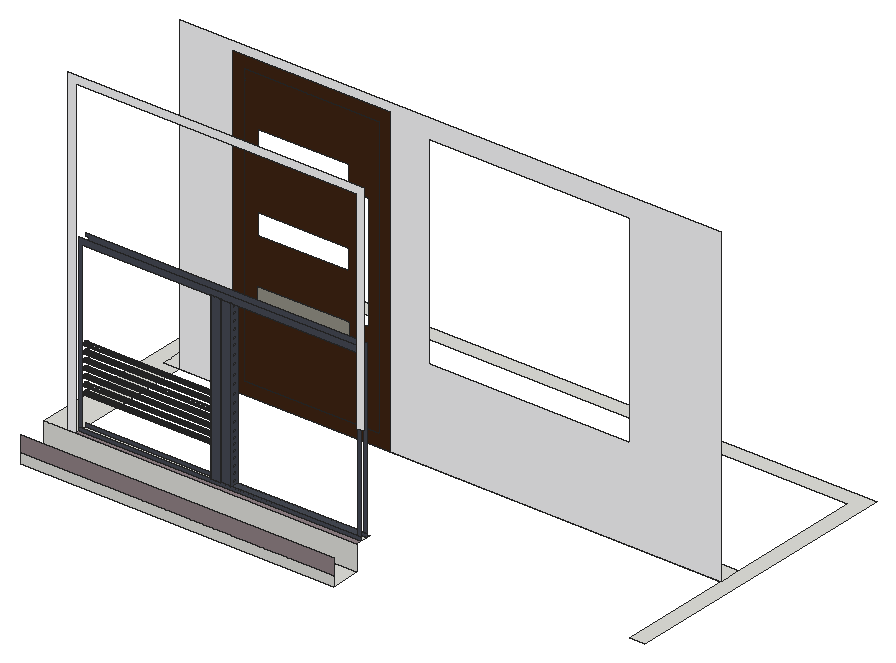
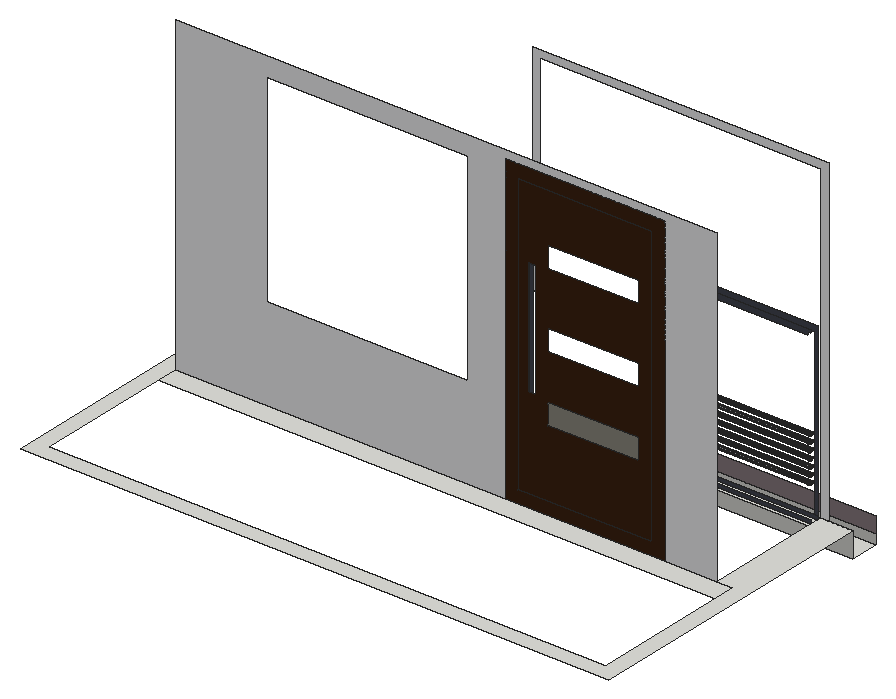
# SketchUp Ruby script. Lengths in inches.
U = 1.inch
M = Sketchup.active_model
def pt(a) = Geom::Point3d.new(a.map { |v| v * U })
def face(e, loops, mat)
  f = e.add_face(loops[0].map { |a| pt(a) })
  loops[1..].each { |l| e.add_face(l.map { |a| pt(a) }).erase! }
  f.material = f.back_material = mat if mat
  f
end
# faces: each face lists its corners as indices into pts; further lists are holes
def faces(e, pts, list, mat = nil) = list.each { |f| face(e, (f[0].is_a?(Array) ? f : [f]).map { |l| l.map { |i| pts[i] } }, mat) }
# xy, xz, yz: faces in a plane at the given z, y or x. An outline is a flat list of corners, or four numbers for a rectangle; further outlines are holes
def ring(l) = l.size == 4 ? [[l[0], l[1]], [l[2], l[1]], [l[2], l[3]], [l[0], l[3]]] : l.each_slice(2).to_a
def flat(e, list, mat, &to3) = list.each { |f| face(e, (f[0].is_a?(Array) ? f : [f]).map { |l| ring(l).map { |u, v| to3.(u, v) } }, mat) }
def xy(e, z, list, mat = nil) = flat(e, list, mat) { |x, y| [x, y, z] }
def xz(e, y, list, mat = nil) = flat(e, list, mat) { |x, z| [x, y, z] }
def yz(e, x, list, mat = nil) = flat(e, list, mat) { |y, z| [x, y, z] }
def lines(e, pts, list) = list.each { |a, b| e.add_line(pt(pts[a]), pt(pts[b])) }
# prism: a flat outline (further loops are holes) pulled along v
def prism(e, loops, v, mat = nil)
  f = face(e, loops, mat); d = Geom::Vector3d.new(v.map { |x| x * U })
  f.pushpull(f.normal.samedirection?(d) ? d.length : -d.length)
end
def box(e, o, s, mat = nil) = prism(e, [[o, [o[0] + s[0], o[1], o[2]], [o[0] + s[0], o[1] + s[1], o[2]], [o[0], o[1] + s[1], o[2]]]], [0, 0, s[2]], mat)
def at(x, y, z, deg = 0) = Geom::Transformation.translation(pt([x, y, z])) * Geom::Transformation.rotation(ORIGIN, Z_AXIS, deg.degrees)
def axes(o, x, y, z) = Geom::Transformation.new([*x, 0, *y, 0, *z, 0, *pt(o).to_a, 1])
def part(name) = M.definitions.add(name)
# library, detail: a bought-in or finely detailed component or shape, given as its bounding box
def library(name, o, s) = part(name).tap { |d| box(d.entities, o, s) }
def detail(e, o, s) = box(e.add_group.entities, o, s)
def put(e, d, t, mat = nil) = e.add_instance(d, t).tap { |i| i.material = mat if mat }
def group(e, t, mat = nil) = e.add_group.tap { |g| g.transformation = t; g.material = mat if mat }.entities
root = M.entities
M.materials.add("[Asphalt New]").color = [145, 130, 134]
M.materials.add("[Formica Graystone]").color = [149, 146, 135]
M.materials.add("[Formica Laminate Dark]").color = [70, 74, 84]
M.materials.add("[Polished Concrete New]").color = [200, 200, 203]
M.materials.add("[Quartz Light Grey]").color = [251, 251, 252]
M.materials.add("[Wood Veneer 01]").color = [63, 37, 19]
xy(root,0,[[96.16,107.04,205.34,117.35]])
xy(root,9,[[96.16,117.35,96.16,223.51,301.48,223.51,301.48,122.78,296.05,122.78,296.05,218.08,101.58,218.08,101.58,162.72,107.21,162.72,107.21,117.35],[107.21,118.87,205.34,121.64],[107.21,121.64,205.34,122.78],[101.58,162.72,296.05,170.43]])
xy(root,9,[[107.21,117.35,205.34,118.87]],"[Asphalt New]")
xy(root,10.25,[[153.22,118.87,156.73,121.64],[156.73,118.87,160.24,121.64]])
xy(root,10.25,[[160.24,118.87,204.4,121.64]],"[Formica Laminate Dark]")
xz(root,107.04,[[96.16,0,205.34,3.4375]])
xz(root,107.04,[[96.16,3.4375,205.34,9]],"[Asphalt New]")
xz(root,117.35,[[96.16,0,205.34,9]])
xz(root,117.35,[[104.33,9,107.21,9,107.21,118.16,205.34,118.16,205.34,44.875,207.77,44.875,207.77,120.875,104.33,120.875]],"[Quartz Light Grey]")
xz(root,118.87,[[107.21,9,205.34,10.25],[107.21,10.25,108.27,10.25,108.27,67.58,204.4,67.58,204.4,10.25,205.34,10.25,205.34,69.75,107.21,69.75],[153.22,10.25,156.73,67.58],[156.73,10.25,160.24,67.58]],"[Formica Laminate Dark]")
xz(root,121.64,[[107.21,9,205.34,10.25],[204.4,10.25,204.4,67.58,108.27,67.58,108.27,68.58,107.21,68.58,107.21,69.75,205.34,69.75,205.34,10.25],[153.22,10.25,156.73,67.58],[156.73,10.25,160.24,67.58]],"[Formica Laminate Dark]")
xz(root,162.72,[[134.59,37.07,166.02,44.51]],"[Formica Graystone]")
xz(root,162.72,[[[107.21,9,125.4,9,125.4,115.21,180.97,115.21,180.97,9,296.05,9,296.05,118.16,107.21,118.16],[194.0625,41.16,264.3125,111.41]]],"[Quartz Light Grey]")
xz(root,162.72,[[[125.4,9,180.97,115.21],[129.81,13.41,176.5625,110.8]],[[129.81,13.41,176.5625,110.8],[134.59,86.26,166.02,93.7],[134.59,60.26,166.02,67.7],[134.59,37.07,166.02,44.51],[170.43,45.29,173.12,85.79]]],"[Wood Veneer 01]")
yz(root,153.22,[[[118.87,10.25,121.64,67.58],[120.22,15.04,120.38,15.06,120.53,15.12,120.66,15.22,120.76,15.35,120.82,15.5,120.84,15.66,120.82,15.82,120.76,15.97,120.66,16.1,120.53,16.2,120.38,16.26,120.22,16.29,120.06,16.26,119.91,16.2,119.78,16.1,119.68,15.97,119.61,15.82,119.59,15.66,119.61,15.5,119.68,15.35,119.78,15.22,119.91,15.12,120.06,15.06],[120.22,65.6,120.38,65.62,120.53,65.68,120.66,65.78,120.76,65.91,120.82,66.0625,120.84,66.22,120.82,66.38,120.76,66.54,120.66,66.66,120.53,66.76,120.38,66.83,120.22,66.85,120.06,66.83,119.91,66.76,119.78,66.66,119.68,66.54,119.61,66.38,119.59,66.22,119.61,66.0625,119.68,65.91,119.78,65.78,119.91,65.68,120.06,65.62],[120.22,63.72,120.38,63.74,120.53,63.81,120.66,63.91,120.76,64.04,120.82,64.1875,120.84,64.35,120.82,64.51,120.76,64.66,120.66,64.79,120.53,64.89,120.38,64.95,120.22,64.97,120.06,64.95,119.91,64.89,119.78,64.79,119.68,64.66,119.61,64.51,119.59,64.35,119.61,64.1875,119.68,64.04,119.78,63.91,119.91,63.81,120.06,63.74],[120.22,61.16,120.38,61.18,120.53,61.24,120.66,61.34,120.76,61.47,120.82,61.625,120.84,61.79,120.82,61.95,120.76,62.1,120.66,62.23,120.53,62.33,120.38,62.39,120.22,62.41,120.06,62.39,119.91,62.33,119.78,62.23,119.68,62.1,119.61,61.95,119.59,61.79,119.61,61.625,119.68,61.47,119.78,61.34,119.91,61.24,120.06,61.18],[120.22,58.6,120.38,58.62,120.53,58.68,120.66,58.78,120.76,58.91,120.82,59.0625,120.84,59.22,120.82,59.38,120.76,59.54,120.66,59.66,120.53,59.76,120.38,59.83,120.22,59.85,120.06,59.83,119.91,59.76,119.78,59.66,119.68,59.54,119.61,59.38,119.59,59.22,119.61,59.0625,119.68,58.91,119.78,58.78,119.91,58.68,120.06,58.62],[120.22,56.04,120.38,56.06,120.53,56.12,120.66,56.22,120.76,56.35,120.82,56.5,120.84,56.66,120.82,56.82,120.76,56.97,120.66,57.1,120.53,57.2,120.38,57.26,120.22,57.29,120.06,57.26,119.91,57.2,119.78,57.1,119.68,56.97,119.61,56.82,119.59,56.66,119.61,56.5,119.68,56.35,119.78,56.22,119.91,56.12,120.06,56.06],[120.22,53.47,120.38,53.49,120.53,53.56,120.66,53.66,120.76,53.79,120.82,53.9375,120.84,54.1,120.82,54.26,120.76,54.41,120.66,54.54,120.53,54.64,120.38,54.7,120.22,54.72,120.06,54.7,119.91,54.64,119.78,54.54,119.68,54.41,119.61,54.26,119.59,54.1,119.61,53.9375,119.68,53.79,119.78,53.66,119.91,53.56,120.06,53.49],[120.22,50.91,120.38,50.93,120.53,50.99,120.66,51.09,120.76,51.22,120.82,51.375,120.84,51.54,120.82,51.7,120.76,51.85,120.66,51.98,120.53,52.08,120.38,52.14,120.22,52.16,120.06,52.14,119.91,52.08,119.78,51.98,119.68,51.85,119.61,51.7,119.59,51.54,119.61,51.375,119.68,51.22,119.78,51.09,119.91,50.99,120.06,50.93],[120.22,48.35,120.38,48.37,120.53,48.43,120.66,48.53,120.76,48.66,120.82,48.8125,120.84,48.97,120.82,49.13,120.76,49.29,120.66,49.41,120.53,49.51,120.38,49.58,120.22,49.6,120.06,49.58,119.91,49.51,119.78,49.41,119.68,49.29,119.61,49.13,119.59,48.97,119.61,48.8125,119.68,48.66,119.78,48.53,119.91,48.43,120.06,48.37],[120.22,45.79,120.38,45.81,120.53,45.87,120.66,45.97,120.76,46.1,120.82,46.25,120.84,46.41,120.82,46.57,120.76,46.72,120.66,46.85,120.53,46.95,120.38,47.01,120.22,47.04,120.06,47.01,119.91,46.95,119.78,46.85,119.68,46.72,119.61,46.57,119.59,46.41,119.61,46.25,119.68,46.1,119.78,45.97,119.91,45.87,120.06,45.81],[120.22,43.22,120.38,43.24,120.53,43.31,120.66,43.41,120.76,43.54,120.82,43.6875,120.84,43.85,120.82,44.01,120.76,44.16,120.66,44.29,120.53,44.39,120.38,44.45,120.22,44.47,120.06,44.45,119.91,44.39,119.78,44.29,119.68,44.16,119.61,44.01,119.59,43.85,119.61,43.6875,119.68,43.54,119.78,43.41,119.91,43.31,120.06,43.24],[120.22,40.66,120.38,40.68,120.53,40.74,120.66,40.84,120.76,40.97,120.82,41.125,120.84,41.29,120.82,41.45,120.76,41.6,120.66,41.73,120.53,41.83,120.38,41.89,120.22,41.91,120.06,41.89,119.91,41.83,119.78,41.73,119.68,41.6,119.61,41.45,119.59,41.29,119.61,41.125,119.68,40.97,119.78,40.84,119.91,40.74,120.06,40.68],[120.22,38.1,120.38,38.12,120.53,38.18,120.66,38.28,120.76,38.41,120.82,38.5625,120.84,38.72,120.82,38.88,120.76,39.04,120.66,39.16,120.53,39.26,120.38,39.33,120.22,39.35,120.06,39.33,119.91,39.26,119.78,39.16,119.68,39.04,119.61,38.88,119.59,38.72,119.61,38.5625,119.68,38.41,119.78,38.28,119.91,38.18,120.06,38.12],[120.22,35.54,120.38,35.56,120.53,35.62,120.66,35.72,120.76,35.85,120.82,36,120.84,36.16,120.82,36.32,120.76,36.47,120.66,36.6,120.53,36.7,120.38,36.76,120.22,36.79,120.06,36.76,119.91,36.7,119.78,36.6,119.68,36.47,119.61,36.32,119.59,36.16,119.61,36,119.68,35.85,119.78,35.72,119.91,35.62,120.06,35.56],[120.22,32.97,120.38,32.99,120.53,33.06,120.66,33.16,120.76,33.29,120.82,33.4375,120.84,33.6,120.82,33.76,120.76,33.91,120.66,34.04,120.53,34.14,120.38,34.2,120.22,34.22,120.06,34.2,119.91,34.14,119.78,34.04,119.68,33.91,119.61,33.76,119.59,33.6,119.61,33.4375,119.68,33.29,119.78,33.16,119.91,33.06,120.06,32.99],[120.22,30.41,120.38,30.43,120.53,30.49,120.66,30.59,120.76,30.72,120.82,30.875,120.84,31.04,120.82,31.2,120.76,31.35,120.66,31.48,120.53,31.58,120.38,31.64,120.22,31.66,120.06,31.64,119.91,31.58,119.78,31.48,119.68,31.35,119.61,31.2,119.59,31.04,119.61,30.875,119.68,30.72,119.78,30.59,119.91,30.49,120.06,30.43],[120.22,27.85,120.38,27.87,120.53,27.93,120.66,28.03,120.76,28.16,120.82,28.3125,120.84,28.47,120.82,28.63,120.76,28.79,120.66,28.91,120.53,29.01,120.38,29.08,120.22,29.1,120.06,29.08,119.91,29.01,119.78,28.91,119.68,28.79,119.61,28.63,119.59,28.47,119.61,28.3125,119.68,28.16,119.78,28.03,119.91,27.93,120.06,27.87],[120.22,25.29,120.38,25.31,120.53,25.37,120.66,25.47,120.76,25.6,120.82,25.75,120.84,25.91,120.82,26.07,120.76,26.22,120.66,26.35,120.53,26.45,120.38,26.51,120.22,26.54,120.06,26.51,119.91,26.45,119.78,26.35,119.68,26.22,119.61,26.07,119.59,25.91,119.61,25.75,119.68,25.6,119.78,25.47,119.91,25.37,120.06,25.31],[120.22,22.72,120.38,22.74,120.53,22.81,120.66,22.91,120.76,23.04,120.82,23.1875,120.84,23.35,120.82,23.51,120.76,23.66,120.66,23.79,120.53,23.89,120.38,23.95,120.22,23.97,120.06,23.95,119.91,23.89,119.78,23.79,119.68,23.66,119.61,23.51,119.59,23.35,119.61,23.1875,119.68,23.04,119.78,22.91,119.91,22.81,120.06,22.74],[120.22,20.16,120.38,20.18,120.53,20.24,120.66,20.34,120.76,20.47,120.82,20.625,120.84,20.79,120.82,20.95,120.76,21.1,120.66,21.23,120.53,21.33,120.38,21.39,120.22,21.41,120.06,21.39,119.91,21.33,119.78,21.23,119.68,21.1,119.61,20.95,119.59,20.79,119.61,20.625,119.68,20.47,119.78,20.34,119.91,20.24,120.06,20.18],[120.22,17.6,120.38,17.62,120.53,17.68,120.66,17.78,120.76,17.91,120.82,18.0625,120.84,18.22,120.82,18.38,120.76,18.54,120.66,18.66,120.53,18.76,120.38,18.83,120.22,18.85,120.06,18.83,119.91,18.76,119.78,18.66,119.68,18.54,119.61,18.38,119.59,18.22,119.61,18.0625,119.68,17.91,119.78,17.78,119.91,17.68,120.06,17.62],[120.22,10.47,120.38,10.49,120.53,10.56,120.66,10.66,120.76,10.79,120.82,10.9375,120.84,11.1,120.82,11.26,120.76,11.41,120.66,11.54,120.53,11.64,120.38,11.7,120.22,11.72,120.06,11.7,119.91,11.64,119.78,11.54,119.68,11.41,119.61,11.26,119.59,11.1,119.61,10.9375,119.68,10.79,119.78,10.66,119.91,10.56,120.06,10.49],[120.22,12.47,120.38,12.49,120.53,12.56,120.66,12.66,120.76,12.79,120.82,12.9375,120.84,13.1,120.82,13.26,120.76,13.41,120.66,13.54,120.53,13.64,120.38,13.7,120.22,13.72,120.06,13.7,119.91,13.64,119.78,13.54,119.68,13.41,119.61,13.26,119.59,13.1,119.61,12.9375,119.68,12.79,119.78,12.66,119.91,12.56,120.06,12.49]]],"[Formica Laminate Dark]")
yz(root,156.73,[[118.87,10.25,121.64,67.58]])
yz(root,160.24,[[[118.87,10.25,121.64,67.58],[120.29,15.54,120.13,15.5625,119.98,15.625,119.85,15.72,119.75,15.85,119.6875,16,119.66,16.16,119.6875,16.33,119.75,16.48,119.85,16.61,119.98,16.71,120.13,16.77,120.29,16.79,120.45,16.77,120.6,16.71,120.73,16.61,120.83,16.48,120.89,16.33,120.91,16.16,120.89,16,120.83,15.85,120.73,15.72,120.6,15.625,120.45,15.5625],[120.29,63.23,120.13,63.25,119.98,63.3125,119.85,63.41,119.75,63.54,119.6875,63.69,119.66,63.85,119.6875,64.01,119.75,64.16,119.85,64.29,119.98,64.39,120.13,64.46,120.29,64.48,120.45,64.46,120.6,64.39,120.73,64.29,120.83,64.16,120.89,64.01,120.91,63.85,120.89,63.69,120.83,63.54,120.73,63.41,120.6,63.3125,120.45,63.25],[120.29,65.54,120.13,65.5625,119.98,65.625,119.85,65.72,119.75,65.85,119.6875,66,119.66,66.16,119.6875,66.33,119.75,66.48,119.85,66.61,119.98,66.71,120.13,66.77,120.29,66.79,120.45,66.77,120.6,66.71,120.73,66.61,120.83,66.48,120.89,66.33,120.91,66.16,120.89,66,120.83,65.85,120.73,65.72,120.6,65.625,120.45,65.5625],[120.29,60.85,120.13,60.875,119.98,60.9375,119.85,61.04,119.75,61.16,119.6875,61.32,119.66,61.48,119.6875,61.64,119.75,61.79,119.85,61.92,119.98,62.02,120.13,62.08,120.29,62.1,120.45,62.08,120.6,62.02,120.73,61.92,120.83,61.79,120.89,61.64,120.91,61.48,120.89,61.32,120.83,61.16,120.73,61.04,120.6,60.9375,120.45,60.875],[120.29,58.16,120.13,58.1875,119.98,58.25,119.85,58.35,119.75,58.48,119.6875,58.63,119.66,58.79,119.6875,58.95,119.75,59.1,119.85,59.23,119.98,59.33,120.13,59.39,120.29,59.41,120.45,59.39,120.6,59.33,120.73,59.23,120.83,59.1,120.89,58.95,120.91,58.79,120.89,58.63,120.83,58.48,120.73,58.35,120.6,58.25,120.45,58.1875],[120.29,55.6,120.13,55.625,119.98,55.6875,119.85,55.79,119.75,55.91,119.6875,56.07,119.66,56.23,119.6875,56.39,119.75,56.54,119.85,56.67,119.98,56.77,120.13,56.83,120.29,56.85,120.45,56.83,120.6,56.77,120.73,56.67,120.83,56.54,120.89,56.39,120.91,56.23,120.89,56.07,120.83,55.91,120.73,55.79,120.6,55.6875,120.45,55.625],[120.29,53.35,120.13,53.375,119.98,53.4375,119.85,53.54,119.75,53.66,119.6875,53.82,119.66,53.98,119.6875,54.14,119.75,54.29,119.85,54.42,119.98,54.52,120.13,54.58,120.29,54.6,120.45,54.58,120.6,54.52,120.73,54.42,120.83,54.29,120.89,54.14,120.91,53.98,120.89,53.82,120.83,53.66,120.73,53.54,120.6,53.4375,120.45,53.375],[120.29,50.29,120.13,50.3125,119.98,50.375,119.85,50.47,119.75,50.6,119.6875,50.75,119.66,50.91,119.6875,51.08,119.75,51.23,119.85,51.36,119.98,51.46,120.13,51.52,120.29,51.54,120.45,51.52,120.6,51.46,120.73,51.36,120.83,51.23,120.89,51.08,120.91,50.91,120.89,50.75,120.83,50.6,120.73,50.47,120.6,50.375,120.45,50.3125],[120.29,47.41,120.13,47.4375,119.98,47.5,119.85,47.6,119.75,47.73,119.6875,47.88,119.66,48.04,119.6875,48.2,119.75,48.35,119.85,48.48,119.98,48.58,120.13,48.64,120.29,48.66,120.45,48.64,120.6,48.58,120.73,48.48,120.83,48.35,120.89,48.2,120.91,48.04,120.89,47.88,120.83,47.73,120.73,47.6,120.6,47.5,120.45,47.4375],[120.29,43.91,120.13,43.9375,119.98,44,119.85,44.1,119.75,44.23,119.6875,44.38,119.66,44.54,119.6875,44.7,119.75,44.85,119.85,44.98,119.98,45.08,120.13,45.14,120.29,45.16,120.45,45.14,120.6,45.08,120.73,44.98,120.83,44.85,120.89,44.7,120.91,44.54,120.89,44.38,120.83,44.23,120.73,44.1,120.6,44,120.45,43.9375],[120.29,41.04,120.13,41.0625,119.98,41.125,119.85,41.22,119.75,41.35,119.6875,41.5,119.66,41.66,119.6875,41.83,119.75,41.98,119.85,42.11,119.98,42.21,120.13,42.27,120.29,42.29,120.45,42.27,120.6,42.21,120.73,42.11,120.83,41.98,120.89,41.83,120.91,41.66,120.89,41.5,120.83,41.35,120.73,41.22,120.6,41.125,120.45,41.0625],[120.29,38.04,120.13,38.0625,119.98,38.125,119.85,38.22,119.75,38.35,119.6875,38.5,119.66,38.66,119.6875,38.83,119.75,38.98,119.85,39.11,119.98,39.21,120.13,39.27,120.29,39.29,120.45,39.27,120.6,39.21,120.73,39.11,120.83,38.98,120.89,38.83,120.91,38.66,120.89,38.5,120.83,38.35,120.73,38.22,120.6,38.125,120.45,38.0625],[120.29,35.29,120.13,35.3125,119.98,35.375,119.85,35.47,119.75,35.6,119.6875,35.75,119.66,35.91,119.6875,36.08,119.75,36.23,119.85,36.36,119.98,36.46,120.13,36.52,120.29,36.54,120.45,36.52,120.6,36.46,120.73,36.36,120.83,36.23,120.89,36.08,120.91,35.91,120.89,35.75,120.83,35.6,120.73,35.47,120.6,35.375,120.45,35.3125],[120.29,32.16,120.13,32.1875,119.98,32.25,119.85,32.35,119.75,32.48,119.6875,32.63,119.66,32.79,119.6875,32.95,119.75,33.1,119.85,33.23,119.98,33.33,120.13,33.39,120.29,33.41,120.45,33.39,120.6,33.33,120.73,33.23,120.83,33.1,120.89,32.95,120.91,32.79,120.89,32.63,120.83,32.48,120.73,32.35,120.6,32.25,120.45,32.1875],[120.29,29.35,120.13,29.375,119.98,29.4375,119.85,29.54,119.75,29.66,119.6875,29.82,119.66,29.98,119.6875,30.14,119.75,30.29,119.85,30.42,119.98,30.52,120.13,30.58,120.29,30.6,120.45,30.58,120.6,30.52,120.73,30.42,120.83,30.29,120.89,30.14,120.91,29.98,120.89,29.82,120.83,29.66,120.73,29.54,120.6,29.4375,120.45,29.375],[120.29,26.41,120.13,26.4375,119.98,26.5,119.85,26.6,119.75,26.73,119.6875,26.88,119.66,27.04,119.6875,27.2,119.75,27.35,119.85,27.48,119.98,27.58,120.13,27.64,120.29,27.66,120.45,27.64,120.6,27.58,120.73,27.48,120.83,27.35,120.89,27.2,120.91,27.04,120.89,26.88,120.83,26.73,120.73,26.6,120.6,26.5,120.45,26.4375],[120.29,24.23,120.13,24.25,119.98,24.3125,119.85,24.41,119.75,24.54,119.6875,24.69,119.66,24.85,119.6875,25.01,119.75,25.16,119.85,25.29,119.98,25.39,120.13,25.46,120.29,25.48,120.45,25.46,120.6,25.39,120.73,25.29,120.83,25.16,120.89,25.01,120.91,24.85,120.89,24.69,120.83,24.54,120.73,24.41,120.6,24.3125,120.45,24.25],[120.29,22.48,120.13,22.5,119.98,22.5625,119.85,22.66,119.75,22.79,119.6875,22.94,119.66,23.1,119.6875,23.26,119.75,23.41,119.85,23.54,119.98,23.64,120.13,23.71,120.29,23.73,120.45,23.71,120.6,23.64,120.73,23.54,120.83,23.41,120.89,23.26,120.91,23.1,120.89,22.94,120.83,22.79,120.73,22.66,120.6,22.5625,120.45,22.5],[120.29,20.29,120.13,20.3125,119.98,20.375,119.85,20.47,119.75,20.6,119.6875,20.75,119.66,20.91,119.6875,21.08,119.75,21.23,119.85,21.36,119.98,21.46,120.13,21.52,120.29,21.54,120.45,21.52,120.6,21.46,120.73,21.36,120.83,21.23,120.89,21.08,120.91,20.91,120.89,20.75,120.83,20.6,120.73,20.47,120.6,20.375,120.45,20.3125],[120.29,17.91,120.13,17.9375,119.98,18,119.85,18.1,119.75,18.23,119.6875,18.38,119.66,18.54,119.6875,18.7,119.75,18.85,119.85,18.98,119.98,19.08,120.13,19.14,120.29,19.16,120.45,19.14,120.6,19.08,120.73,18.98,120.83,18.85,120.89,18.7,120.91,18.54,120.89,18.38,120.83,18.23,120.73,18.1,120.6,18,120.45,17.9375],[120.29,10.73,120.13,10.75,119.98,10.8125,119.85,10.91,119.75,11.04,119.6875,11.19,119.66,11.35,119.6875,11.51,119.75,11.66,119.85,11.79,119.98,11.89,120.13,11.96,120.29,11.98,120.45,11.96,120.6,11.89,120.73,11.79,120.83,11.66,120.89,11.51,120.91,11.35,120.89,11.19,120.83,11.04,120.73,10.91,120.6,10.8125,120.45,10.75],[120.29,13.16,120.13,13.1875,119.98,13.25,119.85,13.35,119.75,13.48,119.6875,13.63,119.66,13.79,119.6875,13.95,119.75,14.1,119.85,14.23,119.98,14.33,120.13,14.39,120.29,14.41,120.45,14.39,120.6,14.33,120.73,14.23,120.83,14.1,120.89,13.95,120.91,13.79,120.89,13.63,120.83,13.48,120.73,13.35,120.6,13.25,120.45,13.1875]]],"[Formica Laminate Dark]")
p = [[108.27,119.78,20.34],[108.27,119.91,20.24],[153.22,119.91,20.24],[153.22,119.78,20.34],[108.27,120.06,20.18],[153.22,120.06,20.18],
  [108.27,120.38,20.18],[108.27,120.53,20.24],[153.22,120.53,20.24],[153.22,120.38,20.18],[108.27,120.66,20.34],[153.22,120.66,20.34],
  [108.27,119.68,20.47],[153.22,119.68,20.47],[108.27,120.76,20.47],[153.22,120.76,20.47],[108.27,119.61,20.625],[153.22,119.61,20.625],
  [108.27,120.82,20.625],[153.22,120.82,20.625],[108.27,119.59,20.79],[153.22,119.59,20.79],[108.27,120.84,20.79],[153.22,120.84,20.79],
  [108.27,119.61,20.95],[153.22,119.61,20.95],[108.27,120.82,20.95],[153.22,120.82,20.95],[108.27,119.68,21.1],[153.22,119.68,21.1],
  [108.27,120.76,21.1],[153.22,120.76,21.1],[108.27,119.78,21.23],[153.22,119.78,21.23],[108.27,120.66,21.23],[153.22,120.66,21.23],
  [108.27,119.91,21.33],[153.22,119.91,21.33],[108.27,120.53,21.33],[153.22,120.53,21.33],[108.27,120.06,21.39],[153.22,120.06,21.39],
  [108.27,120.38,21.39],[153.22,120.38,21.39],[108.27,120.22,21.41],[153.22,120.22,21.41],[108.27,119.91,22.81],[108.27,120.06,22.74],
  [153.22,120.06,22.74],[153.22,119.91,22.81],[108.27,120.22,22.72],[153.22,120.22,22.72],[108.27,120.38,22.74],[153.22,120.38,22.74],
  [108.27,120.53,22.81],[153.22,120.53,22.81],[108.27,119.78,22.91],[153.22,119.78,22.91],[108.27,120.66,22.91],[153.22,120.66,22.91],
  [108.27,119.68,23.04],[153.22,119.68,23.04],[108.27,120.76,23.04],[153.22,120.76,23.04],[108.27,119.61,23.1875],[153.22,119.61,23.1875],
  [108.27,120.82,23.1875],[153.22,120.82,23.1875],[108.27,119.59,23.35],[153.22,119.59,23.35],[108.27,120.84,23.35],[153.22,120.84,23.35],
  [108.27,119.61,23.51],[153.22,119.61,23.51],[108.27,120.82,23.51],[153.22,120.82,23.51],[108.27,119.68,23.66],[153.22,119.68,23.66],
  [108.27,120.76,23.66],[153.22,120.76,23.66],[108.27,119.78,23.79],[153.22,119.78,23.79],[108.27,120.66,23.79],[153.22,120.66,23.79],
  [108.27,119.91,23.89],[153.22,119.91,23.89],[108.27,120.53,23.89],[153.22,120.53,23.89],[108.27,120.06,23.95],[153.22,120.06,23.95],
  [108.27,120.38,23.95],[153.22,120.38,23.95],[108.27,120.22,23.97],[153.22,120.22,23.97],[108.27,119.91,25.37],[108.27,120.06,25.31],
  [153.22,120.06,25.31],[153.22,119.91,25.37],[108.27,120.22,25.29],[153.22,120.22,25.29],[108.27,120.38,25.31],[153.22,120.38,25.31],
  [108.27,120.53,25.37],[153.22,120.53,25.37],[108.27,119.78,25.47],[153.22,119.78,25.47],[108.27,120.66,25.47],[153.22,120.66,25.47],
  [108.27,119.68,25.6],[153.22,119.68,25.6],[108.27,120.76,25.6],[153.22,120.76,25.6],[108.27,119.61,25.75],[153.22,119.61,25.75],
  [108.27,120.82,25.75],[153.22,120.82,25.75],[108.27,119.59,25.91],[153.22,119.59,25.91],[108.27,120.84,25.91],[153.22,120.84,25.91],
  [108.27,119.61,26.07],[153.22,119.61,26.07],[108.27,120.82,26.07],[153.22,120.82,26.07],[108.27,119.68,26.22],[153.22,119.68,26.22],
  [108.27,120.76,26.22],[153.22,120.76,26.22],[108.27,119.78,26.35],[153.22,119.78,26.35],[108.27,120.66,26.35],[153.22,120.66,26.35],
  [108.27,119.91,26.45],[153.22,119.91,26.45],[108.27,120.53,26.45],[153.22,120.53,26.45],[108.27,120.06,26.51],[153.22,120.06,26.51],
  [108.27,120.22,26.54],[153.22,120.22,26.54],[108.27,120.38,26.51],[153.22,120.38,26.51],[108.27,120.06,27.87],[108.27,120.22,27.85],
  [153.22,120.22,27.85],[153.22,120.06,27.87],[108.27,120.38,27.87],[153.22,120.38,27.87],[108.27,119.78,28.03],[108.27,119.91,27.93],
  [153.22,119.91,27.93],[153.22,119.78,28.03],[108.27,120.53,27.93],[153.22,120.53,27.93],[108.27,120.66,28.03],[153.22,120.66,28.03],
  [108.27,119.68,28.16],[153.22,119.68,28.16],[108.27,120.76,28.16],[153.22,120.76,28.16],[108.27,119.61,28.3125],[153.22,119.61,28.3125],
  [108.27,120.82,28.3125],[153.22,120.82,28.3125],[108.27,119.59,28.47],[153.22,119.59,28.47],[108.27,120.84,28.47],[153.22,120.84,28.47],
  [108.27,119.61,28.63],[153.22,119.61,28.63],[108.27,120.82,28.63],[153.22,120.82,28.63],[108.27,119.68,28.79],[153.22,119.68,28.79],
  [108.27,120.76,28.79],[153.22,120.76,28.79],[108.27,119.78,28.91],[153.22,119.78,28.91],[108.27,120.66,28.91],[153.22,120.66,28.91],
  [108.27,119.91,29.01],[153.22,119.91,29.01],[108.27,120.53,29.01],[153.22,120.53,29.01],[108.27,120.06,29.08],[153.22,120.06,29.08],
  [108.27,120.38,29.08],[153.22,120.38,29.08],[108.27,120.22,29.1],[153.22,120.22,29.1],[108.27,119.91,30.49],[108.27,120.06,30.43],
  [153.22,120.06,30.43],[153.22,119.91,30.49],[108.27,120.22,30.41],[153.22,120.22,30.41],[108.27,120.38,30.43],[153.22,120.38,30.43],
  [108.27,120.53,30.49],[153.22,120.53,30.49],[108.27,119.78,30.59],[153.22,119.78,30.59],[108.27,120.66,30.59],[153.22,120.66,30.59],
  [108.27,119.68,30.72],[153.22,119.68,30.72],[108.27,120.76,30.72],[153.22,120.76,30.72],[108.27,119.61,30.875],[153.22,119.61,30.875],
  [108.27,120.82,30.875],[153.22,120.82,30.875],[108.27,119.59,31.04],[153.22,119.59,31.04],[108.27,120.84,31.04],[153.22,120.84,31.04],
  [108.27,119.61,31.2],[153.22,119.61,31.2],[108.27,120.82,31.2],[153.22,120.82,31.2],[108.27,119.68,31.35],[153.22,119.68,31.35],
  [108.27,120.76,31.35],[153.22,120.76,31.35],[108.27,119.78,31.48],[153.22,119.78,31.48],[108.27,120.66,31.48],[153.22,120.66,31.48],
  [108.27,119.91,31.58],[153.22,119.91,31.58],[108.27,120.53,31.58],[153.22,120.53,31.58],[108.27,120.06,31.64],[153.22,120.06,31.64],
  [108.27,120.22,31.66],[153.22,120.22,31.66],[108.27,120.38,31.64],[153.22,120.38,31.64],[108.27,119.91,33.06],[108.27,120.06,32.99],
  [153.22,120.06,32.99],[153.22,119.91,33.06],[108.27,120.22,32.97],[153.22,120.22,32.97],[108.27,120.38,32.99],[153.22,120.38,32.99],
  [108.27,120.53,33.06],[153.22,120.53,33.06],[108.27,119.78,33.16],[153.22,119.78,33.16],[108.27,120.66,33.16],[153.22,120.66,33.16],
  [108.27,119.68,33.29],[153.22,119.68,33.29],[108.27,120.76,33.29],[153.22,120.76,33.29],[108.27,119.61,33.4375],[153.22,119.61,33.4375],
  [108.27,120.82,33.4375],[153.22,120.82,33.4375],[108.27,119.59,33.6],[153.22,119.59,33.6],[108.27,120.84,33.6],[153.22,120.84,33.6],
  [108.27,119.61,33.76],[153.22,119.61,33.76],[108.27,120.82,33.76],[153.22,120.82,33.76],[108.27,119.68,33.91],[153.22,119.68,33.91],
  [108.27,120.76,33.91],[153.22,120.76,33.91],[108.27,119.78,34.04],[153.22,119.78,34.04],[108.27,120.66,34.04],[153.22,120.66,34.04],
  [108.27,119.91,34.14],[153.22,119.91,34.14],[108.27,120.53,34.14],[153.22,120.53,34.14],[108.27,120.06,34.2],[153.22,120.06,34.2],
  [108.27,120.38,34.2],[153.22,120.38,34.2],[108.27,120.22,34.22],[153.22,120.22,34.22],[108.27,120.06,35.56],[108.27,120.22,35.54],
  [153.22,120.22,35.54],[153.22,120.06,35.56],[108.27,120.38,35.56],[153.22,120.38,35.56],[108.27,119.78,35.72],[108.27,119.91,35.62],
  [153.22,119.91,35.62],[153.22,119.78,35.72],[108.27,120.53,35.62],[153.22,120.53,35.62],[108.27,120.66,35.72],[153.22,120.66,35.72],
  [108.27,119.68,35.85],[153.22,119.68,35.85],[108.27,120.76,35.85],[153.22,120.76,35.85],[108.27,119.61,36],[153.22,119.61,36],
  [108.27,120.82,36],[153.22,120.82,36],[108.27,119.59,36.16],[153.22,119.59,36.16],[108.27,120.84,36.16],[153.22,120.84,36.16],
  [108.27,119.61,36.32],[153.22,119.61,36.32],[108.27,120.82,36.32],[153.22,120.82,36.32],[108.27,119.68,36.47],[153.22,119.68,36.47],
  [108.27,120.76,36.47],[153.22,120.76,36.47],[108.27,119.78,36.6],[153.22,119.78,36.6],[108.27,120.66,36.6],[153.22,120.66,36.6],
  [108.27,119.91,36.7],[153.22,119.91,36.7],[108.27,120.53,36.7],[153.22,120.53,36.7],[108.27,120.06,36.76],[153.22,120.06,36.76],
  [108.27,120.38,36.76],[153.22,120.38,36.76],[108.27,120.22,36.79],[153.22,120.22,36.79]]
faces(root,p,[[0,1,2,3],[1,4,5,2],[6,7,8,9],[7,10,11,8],[12,0,3,13],[10,14,15,11],[16,12,13,17],[14,18,19,15],
  [20,16,17,21],[18,22,23,19],[24,20,21,25],[22,26,27,23],[28,24,25,29],[26,30,31,27],[32,28,29,33],[30,34,35,31],
  [36,32,33,37],[34,38,39,35],[40,36,37,41],[38,42,43,39],[44,40,41,45],[42,44,45,43],[46,47,48,49],[47,50,51,48],
  [50,52,53,51],[52,54,55,53],[56,46,49,57],[54,58,59,55],[60,56,57,61],[58,62,63,59],[64,60,61,65],[62,66,67,63],
  [68,64,65,69],[66,70,71,67],[72,68,69,73],[70,74,75,71],[76,72,73,77],[74,78,79,75],[80,76,77,81],[78,82,83,79],
  [84,80,81,85],[82,86,87,83],[88,84,85,89],[86,90,91,87],[92,88,89,93],[90,92,93,91],[94,95,96,97],[95,98,99,96],
  [98,100,101,99],[100,102,103,101],[104,94,97,105],[102,106,107,103],[108,104,105,109],[106,110,111,107],[112,108,109,113],[110,114,115,111],
  [116,112,113,117],[114,118,119,115],[120,116,117,121],[118,122,123,119],[124,120,121,125],[122,126,127,123],[128,124,125,129],[126,130,131,127],
  [132,128,129,133],[130,134,135,131],[136,132,133,137],[138,136,137,139],[140,138,139,141],[134,140,141,135],[142,143,144,145],[143,146,147,144],
  [148,149,150,151],[149,142,145,150],[146,152,153,147],[152,154,155,153],[156,148,151,157],[154,158,159,155],[160,156,157,161],[158,162,163,159],
  [164,160,161,165],[162,166,167,163],[168,164,165,169],[166,170,171,167],[172,168,169,173],[170,174,175,171],[176,172,173,177],[174,178,179,175],
  [180,176,177,181],[178,182,183,179],[184,180,181,185],[182,186,187,183],[188,184,185,189],[186,188,189,187],[190,191,192,193],[191,194,195,192],
  [194,196,197,195],[196,198,199,197],[200,190,193,201],[198,202,203,199],[204,200,201,205],[202,206,207,203],[208,204,205,209],[206,210,211,207],
  [212,208,209,213],[210,214,215,211],[216,212,213,217],[214,218,219,215],[220,216,217,221],[218,222,223,219],[224,220,221,225],[222,226,227,223],
  [228,224,225,229],[226,230,231,227],[232,228,229,233],[234,232,233,235],[236,234,235,237],[230,236,237,231],[238,239,240,241],[239,242,243,240],
  [242,244,245,243],[244,246,247,245],[248,238,241,249],[246,250,251,247],[252,248,249,253],[250,254,255,251],[256,252,253,257],[254,258,259,255],
  [260,256,257,261],[258,262,263,259],[264,260,261,265],[262,266,267,263],[268,264,265,269],[266,270,271,267],[272,268,269,273],[270,274,275,271],
  [276,272,273,277],[274,278,279,275],[280,276,277,281],[278,282,283,279],[284,280,281,285],[282,284,285,283],[286,287,288,289],[287,290,291,288],
  [292,293,294,295],[293,286,289,294],[290,296,297,291],[296,298,299,297],[300,292,295,301],[298,302,303,299],[304,300,301,305],[302,306,307,303],
  [308,304,305,309],[306,310,311,307],[312,308,309,313],[310,314,315,311],[316,312,313,317],[314,318,319,315],[320,316,317,321],[318,322,323,319],
  [324,320,321,325],[322,326,327,323],[328,324,325,329],[326,330,331,327],[332,328,329,333],[330,332,333,331]],"[Polished Concrete New]")
